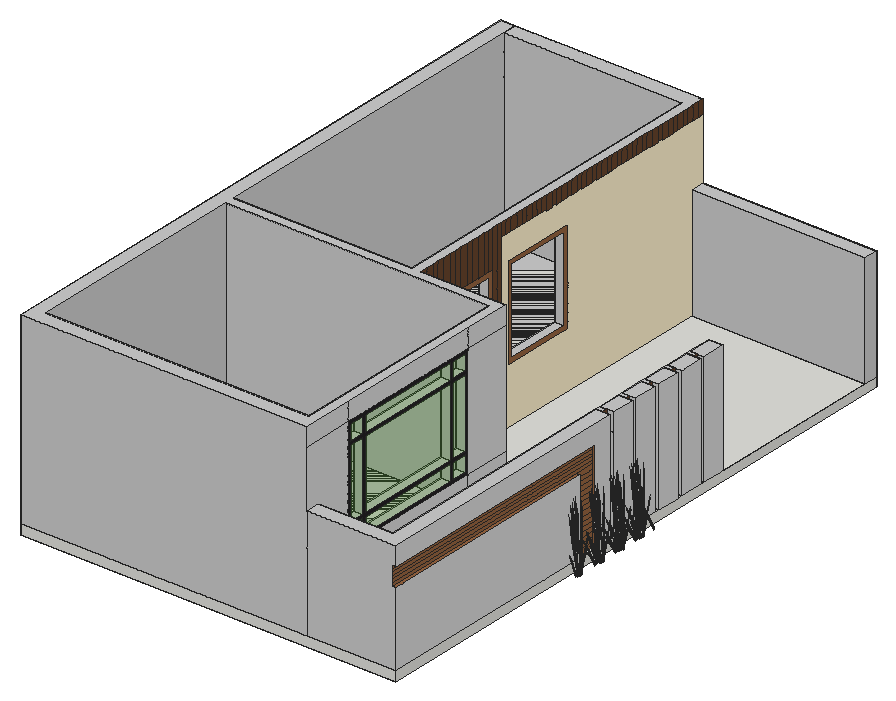
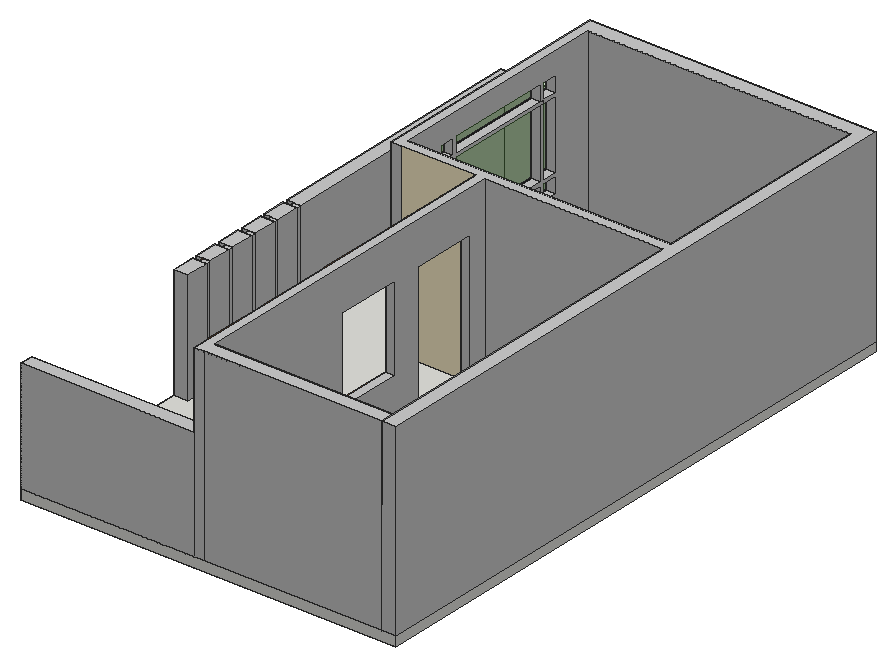
# SketchUp Ruby script. Lengths in inches.
U = 1.inch
M = Sketchup.active_model
def pt(a) = Geom::Point3d.new(a.map { |v| v * U })
def face(e, loops, mat)
  f = e.add_face(loops[0].map { |a| pt(a) })
  loops[1..].each { |l| e.add_face(l.map { |a| pt(a) }).erase! }
  f.material = f.back_material = mat if mat
  f
end
# faces: each face lists its corners as indices into pts; further lists are holes
def faces(e, pts, list, mat = nil) = list.each { |f| face(e, (f[0].is_a?(Array) ? f : [f]).map { |l| l.map { |i| pts[i] } }, mat) }
# xy, xz, yz: faces in a plane at the given z, y or x. An outline is a flat list of corners, or four numbers for a rectangle; further outlines are holes
def ring(l) = l.size == 4 ? [[l[0], l[1]], [l[2], l[1]], [l[2], l[3]], [l[0], l[3]]] : l.each_slice(2).to_a
def flat(e, list, mat, &to3) = list.each { |f| face(e, (f[0].is_a?(Array) ? f : [f]).map { |l| ring(l).map { |u, v| to3.(u, v) } }, mat) }
def xy(e, z, list, mat = nil) = flat(e, list, mat) { |x, y| [x, y, z] }
def xz(e, y, list, mat = nil) = flat(e, list, mat) { |x, z| [x, y, z] }
def yz(e, x, list, mat = nil) = flat(e, list, mat) { |y, z| [x, y, z] }
def lines(e, pts, list) = list.each { |a, b| e.add_line(pt(pts[a]), pt(pts[b])) }
# prism: a flat outline (further loops are holes) pulled along v
def prism(e, loops, v, mat = nil)
  f = face(e, loops, mat); d = Geom::Vector3d.new(v.map { |x| x * U })
  f.pushpull(f.normal.samedirection?(d) ? d.length : -d.length)
end
def box(e, o, s, mat = nil) = prism(e, [[o, [o[0] + s[0], o[1], o[2]], [o[0] + s[0], o[1] + s[1], o[2]], [o[0], o[1] + s[1], o[2]]]], [0, 0, s[2]], mat)
def at(x, y, z, deg = 0) = Geom::Transformation.translation(pt([x, y, z])) * Geom::Transformation.rotation(ORIGIN, Z_AXIS, deg.degrees)
def axes(o, x, y, z) = Geom::Transformation.new([*x, 0, *y, 0, *z, 0, *pt(o).to_a, 1])
def part(name) = M.definitions.add(name)
# library, detail: a bought-in or finely detailed component or shape, given as its bounding box
def library(name, o, s) = part(name).tap { |d| box(d.entities, o, s) }
def detail(e, o, s) = box(e.add_group.entities, o, s)
def put(e, d, t, mat = nil) = e.add_instance(d, t).tap { |i| i.material = mat if mat }
def group(e, t, mat = nil) = e.add_group.tap { |g| g.transformation = t; g.material = mat if mat }.entities
root = M.entities
M.materials.add("D01_Frost_White").color = [255, 242, 206]
M.materials.add("Glass_Basic_01").color = [81, 188, 38]
M.materials["Glass_Basic_01"].alpha = 0.25
M.materials.add("LightPink_Translucent").color = [144, 107, 117]
M.materials["LightPink_Translucent"].alpha = 0.75
M.materials.add("Marble_07_1K").color = [36, 34, 36]
M.materials.add("ThomThom - Waistcoat1").color = [214, 214, 214]
M.materials.add("Wood_Veneer_15_1K").color = [150, 100, 65]
M.materials.add("Wood_Veneer_15_1K1").color = [103, 69, 45]
M.materials.add("wheel_emblem1").color = [204, 204, 204]
c1 = part("blade")
p = [[2.15,0.21,22],[0,0.17,0],[0.09,0.45,0],[2.18,0.31,22],[2.29,0.31,22],[0.38,0.45,0],
  [2.48,0.24,33],[2.49,0.24,33],[2.48,0.22,33]]
faces(c1.entities,p,[[0,1,2,3],[4,5,2,3],[6,3,4,7],[8,0,3,6]])
c2 = part("seeds")
p = [[0.3,-0.1,1.38],[-0.01,-0.03,1.59],[-0.01,-0.03,0.03],[0.14,-0.07,-0.07],[0.29,-0.03,3],[0.15,0.01,3.11]]
faces(c2.entities,p,[[0,1,2,3],[1,0,4,5]],"LightPink_Translucent")
c3 = part("blade with seeds")
put(c3.entities,c1,at(0,0,0))
put(c3.entities,c2,axes([2.4,0.25,30.99],[1.5799,-0.05474,1.17369],[-0.12525,1.92788,0.29478],[-0.07173,-0.02425,1.56792]))
g1 = group(root,at(0,1.43,-6))
box(g1,[0,0,0],[240,384,6])
g2 = group(root,at(0,1.43,0),"wheel_emblem1")
xy(g2,0,[[9,9,177,153],[9,159,123,375],[231,171,235.5,174],[235.5,171,240,174],[231,189.12,235.5,192.12],
  [235.5,189.12,240,192.12],[231,207.24,235.5,210.24],[235.5,207.24,240,210.24],[231,225.37,235.5,228.37],[235.5,225.37,240,228.37],
  [231,243.49,235.5,246.49],[235.5,243.49,240,246.49],[129,375,240,384]])
xy(g2,3,[[123,171,129,213]])
xy(g2,38,[[177,35,183,45],[177,47,183,115],[177,117,183,127]])
xy(g2,39,[[123,231,129,273]])
xy(g2,48,[[177,35,183,45],[177,47,183,115],[177,117,183,127]])
xy(g2,48,[[238,0,240,147]],"Wood_Veneer_15_1K")
xy(g2,50,[[177,35,183,45],[177,47,183,115],[177,117,183,127]])
xy(g2,60,[[238,0,240,159]],"Wood_Veneer_15_1K")
xy(g2,72,[[183,0,240,0,240,171,231,171,231,9,183,9],[231,171,235.5,174],[231,174,240,189.12],[231,189.12,235.5,192.12],[231,192.12,240,207.24],
  [231,207.24,235.5,210.24],[231,210.24,240,225.37],[231,225.37,235.5,228.37],[231,228.37,240,243.49],[231,243.49,235.5,246.49],
  [231,246.49,240,261.49],[129,375,240,384]])
xy(g2,93,[[123,171,129,213],[123,231,129,273]])
xy(g2,94,[[177,35,183,45],[177,47,183,115],[177,117,183,127]])
xy(g2,96,[[177,35,183,45],[177,47,183,115],[177,117,183,127]])
xy(g2,106,[[177,35,183,45],[177,47,183,115],[177,117,183,127]])
xy(g2,120,[[[0,0,183,0,183,159,129,159,129,384,9,384,9,375,123,375,123,159,9,159,9,384,0,384],[9,9,177,153]]])
xz(g2,0,[[0,0,183,120],[183,0,240,0,240,48,238,48,238,60,240,60,240,72,183,72]],"wheel_emblem1")
xz(g2,9,[[9,0,177,120],[177,0,183,72],[183,0,231,72]])
xz(g2,35,[[177,38,183,48],[177,50,183,94],[177,96,183,106]])
xz(g2,45,[[177,38,183,48],[177,50,183,94],[177,96,183,106]])
xz(g2,47,[[177,38,183,48],[177,50,183,94],[177,96,183,106]])
xz(g2,115,[[177,38,183,48],[177,50,183,94],[177,96,183,106]])
xz(g2,117,[[177,38,183,48],[177,50,183,94],[177,96,183,106]])
xz(g2,127,[[177,38,183,48],[177,50,183,94],[177,96,183,106]])
xz(g2,147,[[238,0,240,48]],"Wood_Veneer_15_1K")
xz(g2,153,[[9,0,177,120]])
xz(g2,159,[[9,0,123,120],[177,0,183,120]])
xz(g2,159,[[129,0,177,120]],"D01_Frost_White")
xz(g2,159,[[238,0,240,60]],"Wood_Veneer_15_1K")
xz(g2,171,[[231,0,235.5,72],[235.5,0,240,72],[123,3,129,93]])
xz(g2,174,[[231,0,235.5,60],[235.5,0,240,60],[231,60,235.5,72],[235.5,60,240,72]])
xz(g2,189.12,[[231,0,235.5,72],[235.5,0,240,72]])
xz(g2,192.12,[[231,0,235.5,72],[235.5,0,240,72]])
xz(g2,207.24,[[231,0,235.5,72],[235.5,0,240,72]])
xz(g2,210.24,[[231,0,235.5,72],[235.5,0,240,72]])
xz(g2,213,[[123,3,129,93]])
xz(g2,225.37,[[231,0,235.5,72],[235.5,0,240,72]])
xz(g2,228.37,[[231,0,235.5,72],[235.5,0,240,72]])
xz(g2,231,[[123,39,129,93]])
xz(g2,243.49,[[231,0,235.5,72],[235.5,0,240,72]])
xz(g2,246.49,[[231,0,235.5,72],[235.5,0,240,72]])
xz(g2,261.49,[[231,0,240,72]])
xz(g2,273,[[123,39,129,93]])
xz(g2,375,[[9,0,123,120],[129,0,240,72]])
xz(g2,384,[[0,0,9,120],[123,0,129,120]])
xz(g2,384,[[9,0,123,120],[129,0,240,72]],"wheel_emblem1")
yz(g2,0,[[0,0,384,120]])
yz(g2,9,[[9,0,153,120],[159,0,375,120],[375,72,384,120]])
yz(g2,123,[[[159,0,375,120],[171,3,213,93],[231,39,273,93]]])
yz(g2,129,[[[223.03,0,375,0,375,72,384,72,384,111,223.03,111],[228,36,276,96]]],"D01_Frost_White")
yz(g2,129,[[168,0,168.15,96],[168.15,0,172.72,0,172.72,3,171,3,171,93,213,93,213,3,209.31,3,209.31,0,216,0,216,96,168.15,96],[172.72,0,177.29,3],[177.29,0,181.87,3],[181.87,0,186.44,3],
  [186.44,0,191.01,3],[191.01,0,195.59,3],[195.59,0,200.16,3],[200.16,0,204.73,3],[204.73,0,209.31,3],
  [[228,36,276,96],[231,39,273,93]]],"Wood_Veneer_15_1K")
yz(g2,129,[[159,0,163.57,120],[163.57,0,168,0,168,96,168.15,96,168.15,120,163.57,120],[216,0,219.61,120],[219.61,0,223.03,120],[168.15,96,172.72,120],
  [172.72,96,177.29,120],[177.29,96,181.87,120],[181.87,96,186.44,120],[186.44,96,191.01,120],[191.01,96,195.59,120],
  [195.59,96,200.16,120],[200.16,96,204.73,120],[204.73,96,209.31,120],[209.31,96,212.87,120],[212.87,96,216,120],
  [223.03,111,227.05,120],[227.05,111,231.07,120],[231.07,111,235.1,120],[235.1,111,239.125,120],[239.125,111,243.15,120],
  [243.15,111,247.17,120],[247.17,111,251.2,120],[251.2,111,255.22,120],[255.22,111,259.25,120],[259.25,111,263.27,120],
  [263.27,111,267.29,120],[267.29,111,271.32,120],[271.32,111,275.34,120],[275.34,111,279.37,120],[279.37,111,283.39,120],
  [283.39,111,287.42,120],[287.42,111,291.44,120],[291.44,111,295.46,120],[295.46,111,299.49,120],[299.49,111,303.51,120],
  [303.51,111,307.54,120],[307.54,111,311.5625,120],[311.5625,111,315.59,120],[315.59,111,319.61,120],[319.61,111,323.63,120],
  [323.63,111,327.66,120],[327.66,111,331.68,120],[331.68,111,335.71,120],[335.71,111,339.73,120],[339.73,111,343.76,120],
  [343.76,111,347.78,120],[347.78,111,351.81,120],[351.81,111,355.83,120],[355.83,111,359.85,120],[359.85,111,363.88,120],
  [363.88,111,367.9,120],[367.9,111,371.93,120],[371.93,111,375.95,120],[375.95,111,379.98,120],[379.98,111,384,120]],"Wood_Veneer_15_1K1")
yz(g2,177,[[[9,0,153,120],[47,50,115,50,115,94,47,94,47,96,115,96,115,106,47,106],[47,38,115,48],[35,50,45,94],[117,50,127,94],[35,96,45,106],[117,96,127,106],[117,38,127,48],[35,38,45,48]]])
yz(g2,183,[[35,38,45,48],[47,38,115,48],[117,38,127,48],[35,50,45,94],[47,50,115,94],
  [117,50,127,94],[35,96,45,106],[47,96,115,106],[117,96,127,106]],"Glass_Basic_01")
yz(g2,183,[[[33,36,129,108],[47,50,115,94],[35,38,35,106,127,106,127,38,47,38,47,48,115,48,115,38,117,38,117,48,127,48,127,50,117,50,117,94,127,94,127,96,117,96,117,106,115,106,115,96,47,96,47,106,45,106,45,96,35,96,35,94,45,94,45,50,35,50,35,48,45,48,45,38]]],"Marble_07_1K")
yz(g2,183,[[9,0,33,36],[33,0,129,36],[129,0,159,36],[9,36,33,36,33,108,0,108,0,72,9,72],[129,36,159,108],
  [0,108,33,120],[33,108,129,120],[129,108,159,120]],"ThomThom - Waistcoat1")
yz(g2,231,[[9,0,171,72],[174,0,189.12,72],[192.12,0,207.24,72],[210.24,0,225.37,72],[228.37,0,243.49,72],
  [246.49,0,261.49,72]])
yz(g2,235.5,[[171,0,174,72],[189.12,0,192.12,72],[207.24,0,210.24,72],[225.37,0,228.37,72],[243.49,0,246.49,72]],"Wood_Veneer_15_1K1")
yz(g2,238,[[147,0,159,3],[147,3,159,6],[147,6,159,9],[147,9,159,12],[147,12,159,15],
  [147,15,159,18],[147,18,159,21],[147,21,159,24],[147,24,159,27],[147,27,159,30],
  [147,30,159,33],[147,33,159,36],[147,36,159,39],[147,39,159,42],[147,42,159,45],
  [147,45,159,48],[0,48,159,50],[0,50,159,52],[0,52,159,54],[0,54,159,56],
  [0,56,159,58],[0,58,159,60]],"Wood_Veneer_15_1K")
yz(g2,240,[[375,0,384,72]])
yz(g2,240,[[0,0,147,48],[159,0,171,0,171,72,0,72,0,60,159,60],[174,0,189.12,72],[192.12,0,207.24,72],[210.24,0,225.37,72],
  [228.37,0,243.49,72],[246.49,0,261.49,72]],"ThomThom - Waistcoat1")
p = [[240,261.49,0],[240,375,0],[177,45,96],[177,45,94],[177,47,96],[177,47,94],
  [240,147,0],[240,159,0]]
lines(g2,p,[[0,1],[2,3],[4,2],[5,3],[6,7]])
put(root,c3,axes([250.27,133.53,1.07],[0.08895,0.05019,1.03788],[0.05733,0.5127,-0.22321],[-0.12083,0.09597,0.44375]))
put(root,c3,axes([250.27,151.17,1.07],[0.08895,0.05019,1.03788],[0.05733,0.5127,-0.22321],[-0.12083,0.09597,0.44375]))
put(root,c3,axes([250.27,167.44,1.07],[0.08895,0.05019,1.03788],[0.05733,0.5127,-0.22321],[-0.12083,0.09597,0.44375]))
put(root,c3,axes([250.27,183.29,1.07],[0.08895,0.05019,1.03788],[0.05733,0.5127,-0.22321],[-0.12083,0.09597,0.44375]))
put(root,c3,axes([250.62,148.6875,1.07],[0.04997,0.17024,1.03788],[-0.11515,0.46273,-0.22321],[-0.11824,-0.1106,0.44375]))
put(root,c3,axes([250.62,164.96,1.07],[0.04997,0.17024,1.03788],[-0.11515,0.46273,-0.22321],[-0.11824,-0.1106,0.44375]))
put(root,c3,axes([250.62,180.81,1.07],[0.04997,0.17024,1.03788],[-0.11515,0.46273,-0.22321],[-0.11824,-0.1106,0.44375]))
put(root,c3,axes([250.44,132.1875,0.28],[0.00649,0.09636,1.27986],[-0.13086,0.50324,-0.19552],[-0.09295,-0.02537,0.218]))
put(root,c3,axes([250.44,149.83,0.28],[0.00649,0.09636,1.27986],[-0.13086,0.50324,-0.19552],[-0.09295,-0.02537,0.218]))
put(root,c3,axes([250.44,166.1,0.28],[0.00649,0.09636,1.27986],[-0.13086,0.50324,-0.19552],[-0.09295,-0.02537,0.218]))
put(root,c3,axes([250.44,181.95,0.28],[0.00649,0.09636,1.27986],[-0.13086,0.50324,-0.19552],[-0.09295,-0.02537,0.218]))
put(root,c3,axes([250.09,134.6,1.2],[0.10667,-0.27712,0.83364],[0.04209,0.43871,0.6125],[-0.07709,0.07855,0.18362]))
put(root,c3,axes([250.09,152.24,1.2],[0.10667,-0.27712,0.83364],[0.04209,0.43871,0.6125],[-0.07709,0.07855,0.18362]))
put(root,c3,axes([250.09,168.51,1.2],[0.10667,-0.27712,0.83364],[0.04209,0.43871,0.6125],[-0.07709,0.07855,0.18362]))
put(root,c3,axes([250.09,184.37,1.2],[0.10667,-0.27712,0.83364],[0.04209,0.43871,0.6125],[-0.07709,0.07855,0.18362]))
put(root,c3,axes([250.37,134.89,0.28],[0.03433,0.06109,1.27986],[0.05822,0.56601,-0.19552],[-0.07609,0.1207,0.218]))
put(root,c3,axes([250.37,152.53,0.28],[0.03433,0.06109,1.27986],[0.05822,0.56601,-0.19552],[-0.07609,0.1207,0.218]))
put(root,c3,axes([250.37,168.8,0.28],[0.03433,0.06109,1.27986],[0.05822,0.56601,-0.19552],[-0.07609,0.1207,0.218]))
put(root,c3,axes([250.37,184.65,0.28],[0.03433,0.06109,1.27986],[0.05822,0.56601,-0.19552],[-0.07609,0.1207,0.218]))
put(root,c3,axes([250.32,149.2,1.2],[0.16341,-0.04375,0.83364],[-0.10366,0.38551,0.6125],[-0.08075,-0.05783,0.18362]))
put(root,c3,axes([250.32,165.47,1.2],[0.16341,-0.04375,0.83364],[-0.10366,0.38551,0.6125],[-0.08075,-0.05783,0.18362]))
put(root,c3,axes([250.32,181.32,1.2],[0.16341,-0.04375,0.83364],[-0.10366,0.38551,0.6125],[-0.08075,-0.05783,0.18362]))
put(root,c3,axes([251.3,133.0625,0.6875],[-0.26625,-0.10025,-0.45255],[0.05619,-0.61836,-0.11877],[-0.07946,-0.07493,0.99892]))
put(root,c3,axes([251.3,150.7,0.6875],[-0.26625,-0.10025,-0.45255],[0.05619,-0.61836,-0.11877],[-0.07946,-0.07493,0.99892]))
put(root,c3,axes([251.3,166.97,0.6875],[-0.26625,-0.10025,-0.45255],[0.05619,-0.61836,-0.11877],[-0.07946,-0.07493,0.99892]))
put(root,c3,axes([251.3,182.83,0.6875],[-0.26625,-0.10025,-0.45255],[0.05619,-0.61836,-0.11877],[-0.07946,-0.07493,0.99892]))
put(root,c3,axes([250.95,134.23,0.66],[-0.23955,-0.30573,-0.36036],[0.14318,-0.54821,0],[-0.05456,-0.06963,1.14313]))
put(root,c3,axes([250.95,151.875,0.66],[-0.23955,-0.30573,-0.36036],[0.14318,-0.54821,0],[-0.05456,-0.06963,1.14313]))
put(root,c3,axes([250.95,168.14,0.66],[-0.23955,-0.30573,-0.36036],[0.14318,-0.54821,0],[-0.05456,-0.06963,1.14313]))
put(root,c3,axes([250.95,184,0.66],[-0.23955,-0.30573,-0.36036],[0.14318,-0.54821,0],[-0.05456,-0.06963,1.14313]))
put(root,c3,axes([250.84,147.32,0.28],[-0.02479,0.08055,1.27986],[-0.25056,0.17367,-0.19552],[-0.06053,-0.15798,0.218]))
put(root,c3,axes([250.84,163.59,0.28],[-0.02479,0.08055,1.27986],[-0.25056,0.17367,-0.19552],[-0.06053,-0.15798,0.218]))
put(root,c3,axes([250.84,179.44,0.28],[-0.02479,0.08055,1.27986],[-0.25056,0.17367,-0.19552],[-0.06053,-0.15798,0.218]))
put(root,c3,axes([250.84,194.43,0.28],[-0.02479,0.08055,1.27986],[-0.25056,0.17367,-0.19552],[-0.06053,-0.15798,0.218]))
put(root,c3,axes([251.09,134.6,0.91],[-0.16003,0.61271,0],[-0.26773,-0.34169,-0.37456],[-0.06098,-0.07782,1.18819]))
put(root,c3,axes([251.09,152.24,0.91],[-0.16003,0.61271,0],[-0.26773,-0.34169,-0.37456],[-0.06098,-0.07782,1.18819]))
put(root,c3,axes([251.09,168.51,0.91],[-0.16003,0.61271,0],[-0.26773,-0.34169,-0.37456],[-0.06098,-0.07782,1.18819]))
put(root,c3,axes([251.09,184.36,0.91],[-0.16003,0.61271,0],[-0.26773,-0.34169,-0.37456],[-0.06098,-0.07782,1.18819]))
put(root,c3,axes([250.8,135.49,1.07],[0.08077,-0.09646,1.03788],[0.19942,0.29084,-0.22321],[-0.05936,0.25166,0.44375]))
put(root,c3,axes([250.8,153.13,1.07],[0.08077,-0.09646,1.03788],[0.19942,0.29084,-0.22321],[-0.05936,0.25166,0.44375]))
put(root,c3,axes([250.8,169.4,1.07],[0.08077,-0.09646,1.03788],[0.19942,0.29084,-0.22321],[-0.05936,0.25166,0.44375]))
put(root,c3,axes([250.8,185.25,1.07],[0.08077,-0.09646,1.03788],[0.19942,0.29084,-0.22321],[-0.05936,0.25166,0.44375]))
put(root,c3,axes([250.6875,147.63,0.74],[-0.07384,0.49928,-0.02825],[-0.22725,-0.15358,-0.1281],[-0.0345,-0.08166,0.42251]))
put(root,c3,axes([250.6875,163.9,0.74],[-0.07384,0.49928,-0.02825],[-0.22725,-0.15358,-0.1281],[-0.0345,-0.08166,0.42251]))
put(root,c3,axes([250.6875,179.75,0.74],[-0.07384,0.49928,-0.02825],[-0.22725,-0.15358,-0.1281],[-0.0345,-0.08166,0.42251]))
put(root,c3,axes([251.03,147,1.07],[-0.0155,0.20002,1.03788],[-0.22659,0.16744,-0.22321],[-0.05297,-0.25854,0.44375]))
put(root,c3,axes([251.03,163.27,1.07],[-0.0155,0.20002,1.03788],[-0.22659,0.16744,-0.22321],[-0.05297,-0.25854,0.44375]))
put(root,c3,axes([251.03,179.12,1.07],[-0.0155,0.20002,1.03788],[-0.22659,0.16744,-0.22321],[-0.05297,-0.25854,0.44375]))
put(root,c3,axes([251.03,194.11,1.07],[-0.0155,0.20002,1.03788],[-0.22659,0.16744,-0.22321],[-0.05297,-0.25854,0.44375]))
put(root,c3,axes([251.6,133.15,1.13],[-0.25843,0.40595,-0.21117],[-0.17185,-0.5736,-0.36291],[-0.06376,-0.05825,1.15913]))
put(root,c3,axes([251.6,150.8,1.13],[-0.25843,0.40595,-0.21117],[-0.17185,-0.5736,-0.36291],[-0.06376,-0.05825,1.15913]))
put(root,c3,axes([251.6,167.07,1.13],[-0.25843,0.40595,-0.21117],[-0.17185,-0.5736,-0.36291],[-0.06376,-0.05825,1.15913]))
put(root,c3,axes([251.6,182.92,1.13],[-0.25843,0.40595,-0.21117],[-0.17185,-0.5736,-0.36291],[-0.06376,-0.05825,1.15913]))
put(root,c3,axes([250.5625,149.91,0.91],[-0.32006,0,0],[0,-0.68339,-0.37456],[0,-0.15565,1.18819]))
put(root,c3,axes([250.5625,166.18,0.91],[-0.32006,0,0],[0,-0.68339,-0.37456],[0,-0.15565,1.18819]))
put(root,c3,axes([250.5625,182.03,0.91],[-0.32006,0,0],[0,-0.68339,-0.37456],[0,-0.15565,1.18819]))
put(root,c3,axes([251.01,134,0.66],[-0.06012,-0.53279,-0.22483],[0.23879,-0.15129,0.22483],[-0.04814,-0.06144,1.00865]))
put(root,c3,axes([251.01,151.65,0.66],[-0.06012,-0.53279,-0.22483],[0.23879,-0.15129,0.22483],[-0.04814,-0.06144,1.00865]))
put(root,c3,axes([251.01,167.92,0.66],[-0.06012,-0.53279,-0.22483],[0.23879,-0.15129,0.22483],[-0.04814,-0.06144,1.00865]))
put(root,c3,axes([251.01,183.77,0.66],[-0.06012,-0.53279,-0.22483],[0.23879,-0.15129,0.22483],[-0.04814,-0.06144,1.00865]))
put(root,c3,axes([251.77,133.6,0.6875],[-0.1724,0.45959,-0.45255],[-0.21416,-0.41674,-0.11877],[-0.06908,0.11465,0.99892]))
put(root,c3,axes([251.77,151.24,0.6875],[-0.1724,0.45959,-0.45255],[-0.21416,-0.41674,-0.11877],[-0.06908,0.11465,0.99892]))
put(root,c3,axes([251.77,167.51,0.6875],[-0.1724,0.45959,-0.45255],[-0.21416,-0.41674,-0.11877],[-0.06908,0.11465,0.99892]))
put(root,c3,axes([251.77,183.36,0.6875],[-0.1724,0.45959,-0.45255],[-0.21416,-0.41674,-0.11877],[-0.06908,0.11465,0.99892]))
put(root,c3,axes([250.8125,149.73,0.88],[-0.23808,0.51407,0.22322],[-0.23822,-0.50866,-0.26485],[-0.00831,-0.14599,1.19671]))
put(root,c3,axes([250.8125,166,0.88],[-0.23808,0.51407,0.22322],[-0.23822,-0.50866,-0.26485],[-0.00831,-0.14599,1.19671]))
put(root,c3,axes([250.8125,181.85,0.88],[-0.23808,0.51407,0.22322],[-0.23822,-0.50866,-0.26485],[-0.00831,-0.14599,1.19671]))
put(root,c3,axes([250.95,146.68,1.2],[0.13352,0.21281,0.83364],[-0.19445,0.12793,0.6125],[-0.0416,-0.16355,0.18362]))
put(root,c3,axes([250.95,162.95,1.2],[0.13352,0.21281,0.83364],[-0.19445,0.12793,0.6125],[-0.0416,-0.16355,0.18362]))
put(root,c3,axes([250.95,178.8,1.2],[0.13352,0.21281,0.83364],[-0.19445,0.12793,0.6125],[-0.0416,-0.16355,0.18362]))
put(root,c3,axes([250.95,193.79,1.2],[0.13352,0.21281,0.83364],[-0.19445,0.12793,0.6125],[-0.0416,-0.16355,0.18362]))
put(root,c3,axes([251.89,133.34,0.98],[-0.24993,-0.49214,-0.18284],[0.21031,-0.55263,0.40012],[-0.0673,0.05757,1.22088]))
put(root,c3,axes([251.89,150.98,0.98],[-0.24993,-0.49214,-0.18284],[0.21031,-0.55263,0.40012],[-0.0673,0.05757,1.22088]))
put(root,c3,axes([251.89,167.25,0.98],[-0.24993,-0.49214,-0.18284],[0.21031,-0.55263,0.40012],[-0.0673,0.05757,1.22088]))
put(root,c3,axes([251.89,183.1,0.98],[-0.24993,-0.49214,-0.18284],[0.21031,-0.55263,0.40012],[-0.0673,0.05757,1.22088]))
put(root,c3,axes([251.43,150.51,0.8],[-0.15376,-0.51322,-0.32471],[0.2329,-0.3614,0.15627],[-0.04976,-0.0635,1.04254]))
put(root,c3,axes([251.43,166.78,0.8],[-0.15376,-0.51322,-0.32471],[0.2329,-0.3614,0.15627],[-0.04976,-0.0635,1.04254]))
put(root,c3,axes([251.43,182.63,0.8],[-0.15376,-0.51322,-0.32471],[0.2329,-0.3614,0.15627],[-0.04976,-0.0635,1.04254]))
put(root,c3,axes([250.99,135.8125,1.2],[-0.00662,-0.36357,0.83364],[0.16552,0.25931,0.6125],[-0.03255,0.17329,0.18362]))
put(root,c3,axes([250.99,153.45,1.2],[-0.00662,-0.36357,0.83364],[0.16552,0.25931,0.6125],[-0.03255,0.17329,0.18362]))
put(root,c3,axes([250.99,169.72,1.2],[-0.00662,-0.36357,0.83364],[0.16552,0.25931,0.6125],[-0.03255,0.17329,0.18362]))
put(root,c3,axes([250.99,185.57,1.2],[-0.00662,-0.36357,0.83364],[0.16552,0.25931,0.6125],[-0.03255,0.17329,0.18362]))
put(root,c3,axes([251.76,133.23,0.8],[-0.27795,0.03775,-0.32471],[-0.02514,-0.62656,0.15627],[-0.04976,0.0635,1.04254]))
put(root,c3,axes([251.76,150.875,0.8],[-0.27795,0.03775,-0.32471],[-0.02514,-0.62656,0.15627],[-0.04976,0.0635,1.04254]))
put(root,c3,axes([251.76,167.15,0.8],[-0.27795,0.03775,-0.32471],[-0.02514,-0.62656,0.15627],[-0.04976,0.0635,1.04254]))
put(root,c3,axes([251.76,183,0.8],[-0.27795,0.03775,-0.32471],[-0.02514,-0.62656,0.15627],[-0.04976,0.0635,1.04254]))
put(root,c3,axes([251.23,134.28,0.99],[0.23955,0.30573,0.36036],[-0.14318,0.54821,0],[-0.05456,-0.06963,1.14313]))
put(root,c3,axes([251.23,151.92,0.99],[0.23955,0.30573,0.36036],[-0.14318,0.54821,0],[-0.05456,-0.06963,1.14313]))
put(root,c3,axes([251.23,168.19,0.99],[0.23955,0.30573,0.36036],[-0.14318,0.54821,0],[-0.05456,-0.06963,1.14313]))
put(root,c3,axes([251.23,184.04,0.99],[0.23955,0.30573,0.36036],[-0.14318,0.54821,0],[-0.05456,-0.06963,1.14313]))
put(root,c3,axes([251.46,150.8,0.96],[0.06784,-0.72454,-0.17004],[0.32166,0.1263,0.37211],[-0.05621,-0.10006,1.13542]))
put(root,c3,axes([251.46,167.07,0.96],[0.06784,-0.72454,-0.17004],[0.32166,0.1263,0.37211],[-0.05621,-0.10006,1.13542]))
put(root,c3,axes([251.46,182.92,0.96],[0.06784,-0.72454,-0.17004],[0.32166,0.1263,0.37211],[-0.05621,-0.10006,1.13542]))
put(root,c3,axes([251.57,133.33,1.09],[-0.04938,0.54569,0.10509],[-0.24125,-0.09472,-0.30009],[-0.0439,-0.05603,0.91989]))
put(root,c3,axes([251.57,150.97,1.09],[-0.04938,0.54569,0.10509],[-0.24125,-0.09472,-0.30009],[-0.0439,-0.05603,0.91989]))
put(root,c3,axes([251.57,167.24,1.09],[-0.04938,0.54569,0.10509],[-0.24125,-0.09472,-0.30009],[-0.0439,-0.05603,0.91989]))
put(root,c3,axes([251.57,183.09,1.09],[-0.04938,0.54569,0.10509],[-0.24125,-0.09472,-0.30009],[-0.0439,-0.05603,0.91989]))
put(root,c3,axes([252.05,134.85,0.66],[-0.23955,0.30573,-0.36036],[-0.14318,-0.54821,0],[-0.05456,0.06963,1.14313]))
put(root,c3,axes([252.05,152.49,0.66],[-0.23955,0.30573,-0.36036],[-0.14318,-0.54821,0],[-0.05456,0.06963,1.14313]))
put(root,c3,axes([252.05,168.76,0.66],[-0.23955,0.30573,-0.36036],[-0.14318,-0.54821,0],[-0.05456,0.06963,1.14313]))
put(root,c3,axes([252.05,184.61,0.66],[-0.23955,0.30573,-0.36036],[-0.14318,-0.54821,0],[-0.05456,0.06963,1.14313]))
